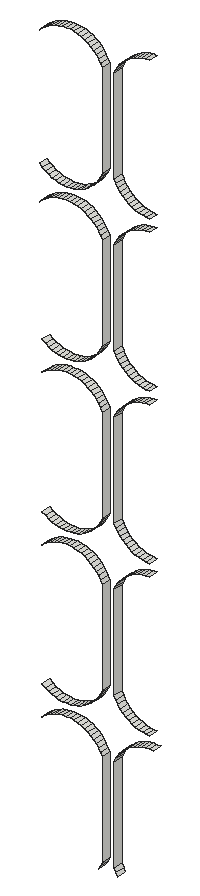
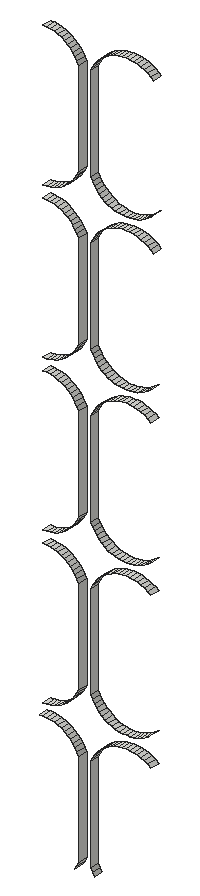
# SketchUp Ruby script. Lengths in inches.
U = 1.inch
M = Sketchup.active_model
def pt(a) = Geom::Point3d.new(a.map { |v| v * U })
def face(e, loops, mat)
  f = e.add_face(loops[0].map { |a| pt(a) })
  loops[1..].each { |l| e.add_face(l.map { |a| pt(a) }).erase! }
  f.material = f.back_material = mat if mat
  f
end
# faces: each face lists its corners as indices into pts; further lists are holes
def faces(e, pts, list, mat = nil) = list.each { |f| face(e, (f[0].is_a?(Array) ? f : [f]).map { |l| l.map { |i| pts[i] } }, mat) }
# xy, xz, yz: faces in a plane at the given z, y or x. An outline is a flat list of corners, or four numbers for a rectangle; further outlines are holes
def ring(l) = l.size == 4 ? [[l[0], l[1]], [l[2], l[1]], [l[2], l[3]], [l[0], l[3]]] : l.each_slice(2).to_a
def flat(e, list, mat, &to3) = list.each { |f| face(e, (f[0].is_a?(Array) ? f : [f]).map { |l| ring(l).map { |u, v| to3.(u, v) } }, mat) }
def xy(e, z, list, mat = nil) = flat(e, list, mat) { |x, y| [x, y, z] }
def xz(e, y, list, mat = nil) = flat(e, list, mat) { |x, z| [x, y, z] }
def yz(e, x, list, mat = nil) = flat(e, list, mat) { |y, z| [x, y, z] }
def lines(e, pts, list) = list.each { |a, b| e.add_line(pt(pts[a]), pt(pts[b])) }
# prism: a flat outline (further loops are holes) pulled along v
def prism(e, loops, v, mat = nil)
  f = face(e, loops, mat); d = Geom::Vector3d.new(v.map { |x| x * U })
  f.pushpull(f.normal.samedirection?(d) ? d.length : -d.length)
end
def box(e, o, s, mat = nil) = prism(e, [[o, [o[0] + s[0], o[1], o[2]], [o[0] + s[0], o[1] + s[1], o[2]], [o[0], o[1] + s[1], o[2]]]], [0, 0, s[2]], mat)
def at(x, y, z, deg = 0) = Geom::Transformation.translation(pt([x, y, z])) * Geom::Transformation.rotation(ORIGIN, Z_AXIS, deg.degrees)
def axes(o, x, y, z) = Geom::Transformation.new([*x, 0, *y, 0, *z, 0, *pt(o).to_a, 1])
def part(name) = M.definitions.add(name)
# library, detail: a bought-in or finely detailed component or shape, given as its bounding box
def library(name, o, s) = part(name).tap { |d| box(d.entities, o, s) }
def detail(e, o, s) = box(e.add_group.entities, o, s)
def put(e, d, t, mat = nil) = e.add_instance(d, t).tap { |i| i.material = mat if mat }
def group(e, t, mat = nil) = e.add_group.tap { |g| g.transformation = t; g.material = mat if mat }.entities
root = M.entities
yz(root,71.5,[[138,52,138.79,60],[138,65,138.79,73],[138,78,138.79,86],[138,91,138.79,99],[138,104,138.79,112]])
yz(root,72.5,[[138,52,138.79,60],[138,65,138.79,73],[138,78,138.79,86],[138,91,138.79,99],[138,104,138.79,112]])
p = [[71.36,138.79,51.71],[71.2,138.79,51.44],[71.2,138,51.44],[71.36,138,51.71],[72.8,138.79,51.44],[72.64,138.79,51.71],
  [72.64,138,51.71],[72.8,138,51.44],[71.5,138.79,52],[71.5,138,52],[72.5,138.79,52],[72.5,138,52],
  [71.36,138.79,60.29],[71.5,138.79,60],[71.5,138,60],[71.36,138,60.29],[72.5,138.79,60],[72.64,138.79,60.29],
  [72.64,138,60.29],[72.5,138,60],[71.2,138.79,60.56],[71.2,138,60.56],[72.8,138.79,60.56],[72.8,138,60.56],
  [71.01,138.79,60.82],[71.01,138,60.82],[72.99,138.79,60.82],[72.99,138,60.82],[70.79,138.79,61.05],[70.79,138,61.05],
  [73.21,138.79,61.05],[73.21,138,61.05],[70.56,138.79,61.26],[70.56,138,61.26],[73.44,138.79,61.26],[73.44,138,61.26],
  [66.44,138.79,61.26],[66.7,138.79,61.45],[66.7,138,61.45],[66.44,138,61.26],[70.3,138.79,61.45],[70.3,138,61.45],
  [73.7,138.79,61.45],[73.7,138,61.45],[66.97,138.79,61.62],[66.97,138,61.62],[70.03,138.79,61.62],[70.03,138,61.62],
  [73.97,138.79,61.62],[73.97,138,61.62],[67.26,138.79,61.75],[67.26,138,61.75],[69.74,138.79,61.75],[69.74,138,61.75],
  [74.26,138.79,61.75],[74.26,138,61.75],[67.56,138.79,61.86],[67.56,138,61.86],[69.44,138.79,61.86],[69.44,138,61.86],
  [74.56,138.79,61.86],[74.56,138,61.86],[67.87,138.79,61.9375],[67.87,138,61.9375],[68.18,138.79,61.98],[68.18,138,61.98],
  [68.82,138.79,61.98],[69.13,138.79,61.9375],[69.13,138,61.9375],[68.82,138,61.98],[74.87,138.79,61.9375],[74.87,138,61.9375],
  [75.18,138.79,61.98],[75.18,138,61.98],[68.5,138.79,62],[68.5,138,62],[75.5,138.79,62],[75.5,138,62],
  [75.82,138.79,61.98],[75.82,138,61.98],[68.18,138.79,63.02],[67.87,138.79,63.0625],[67.87,138,63.0625],[68.18,138,63.02],
  [68.5,138.79,63],[68.5,138,63],[68.82,138.79,63.02],[68.82,138,63.02],[69.13,138.79,63.0625],[69.13,138,63.0625],
  [75.18,138.79,63.02],[74.87,138.79,63.0625],[74.87,138,63.0625],[75.18,138,63.02],[75.5,138.79,63],[75.5,138,63],
  [67.56,138.79,63.14],[67.26,138.79,63.25],[67.26,138,63.25],[67.56,138,63.14],[69.44,138.79,63.14],[69.44,138,63.14],
  [69.74,138.79,63.25],[69.74,138,63.25],[74.56,138.79,63.14],[74.26,138.79,63.25],[74.26,138,63.25],[74.56,138,63.14],
  [66.97,138.79,63.38],[66.97,138,63.38],[70.03,138.79,63.38],[70.03,138,63.38],[73.97,138.79,63.38],[73.97,138,63.38],
  [66.7,138.79,63.55],[66.7,138,63.55],[70.3,138.79,63.55],[70.3,138,63.55],[73.7,138.79,63.55],[73.7,138,63.55],
  [66.44,138.79,63.74],[66.44,138,63.74],[70.56,138.79,63.74],[70.56,138,63.74],[73.44,138.79,63.74],[73.44,138,63.74],
  [70.79,138.79,63.95],[70.79,138,63.95],[73.21,138.79,63.95],[73.21,138,63.95],[71.01,138.79,64.18],[71.01,138,64.18],
  [72.99,138.79,64.18],[72.99,138,64.18],[71.2,138.79,64.44],[71.2,138,64.44],[72.8,138.79,64.44],[72.8,138,64.44],
  [71.36,138.79,64.71],[71.36,138,64.71],[72.64,138.79,64.71],[72.64,138,64.71],[71.5,138.79,65],[71.5,138,65],
  [72.5,138.79,65],[72.5,138,65],[71.36,138.79,73.29],[71.5,138.79,73],[71.5,138,73],[71.36,138,73.29],
  [72.5,138.79,73],[72.64,138.79,73.29],[72.64,138,73.29],[72.5,138,73],[71.2,138.79,73.56],[71.2,138,73.56],
  [72.8,138.79,73.56],[72.8,138,73.56],[71.01,138.79,73.82],[71.01,138,73.82],[72.99,138.79,73.82],[72.99,138,73.82],
  [70.79,138.79,74.05],[70.79,138,74.05],[73.21,138.79,74.05],[73.21,138,74.05],[70.56,138.79,74.26],[70.56,138,74.26],
  [73.44,138.79,74.26],[73.44,138,74.26],[66.44,138.79,74.26],[66.7,138.79,74.45],[66.7,138,74.45],[66.44,138,74.26],
  [70.3,138.79,74.45],[70.3,138,74.45],[73.7,138.79,74.45],[73.7,138,74.45],[66.97,138.79,74.62],[66.97,138,74.62],
  [70.03,138.79,74.62],[70.03,138,74.62],[73.97,138.79,74.62],[73.97,138,74.62],[67.26,138.79,74.75],[67.26,138,74.75],
  [69.74,138.79,74.75],[69.74,138,74.75],[74.26,138.79,74.75],[74.26,138,74.75],[67.56,138.79,74.86],[67.56,138,74.86],
  [69.44,138.79,74.86],[69.44,138,74.86],[74.56,138.79,74.86],[74.56,138,74.86],[67.87,138.79,74.9375],[67.87,138,74.9375],
  [68.18,138.79,74.98],[68.18,138,74.98],[68.82,138.79,74.98],[69.13,138.79,74.9375],[69.13,138,74.9375],[68.82,138,74.98],
  [74.87,138.79,74.9375],[74.87,138,74.9375],[75.18,138.79,74.98],[75.18,138,74.98],[68.5,138.79,75],[68.5,138,75],
  [75.5,138.79,75],[75.5,138,75],[68.18,138.79,76.02],[67.87,138.79,76.0625],[67.87,138,76.0625],[68.18,138,76.02],
  [68.5,138.79,76],[68.5,138,76],[68.82,138.79,76.02],[68.82,138,76.02],[69.13,138.79,76.0625],[69.13,138,76.0625],
  [75.18,138.79,76.02],[74.87,138.79,76.0625],[74.87,138,76.0625],[75.18,138,76.02],[75.5,138.79,76],[75.5,138,76],
  [67.56,138.79,76.14],[67.26,138.79,76.25],[67.26,138,76.25],[67.56,138,76.14],[69.44,138.79,76.14],[69.44,138,76.14],
  [69.74,138.79,76.25],[69.74,138,76.25],[74.56,138.79,76.14],[74.26,138.79,76.25],[74.26,138,76.25],[74.56,138,76.14],
  [66.97,138.79,76.38],[66.97,138,76.38],[70.03,138.79,76.38],[70.03,138,76.38],[73.97,138.79,76.38],[73.97,138,76.38],
  [66.7,138.79,76.55],[66.7,138,76.55],[70.3,138.79,76.55],[70.3,138,76.55],[73.7,138.79,76.55],[73.7,138,76.55],
  [66.44,138.79,76.74],[66.44,138,76.74],[70.56,138.79,76.74],[70.56,138,76.74],[73.44,138.79,76.74],[73.44,138,76.74],
  [70.79,138.79,76.95],[70.79,138,76.95],[73.21,138.79,76.95],[73.21,138,76.95],[71.01,138.79,77.18],[71.01,138,77.18],
  [72.99,138.79,77.18],[72.99,138,77.18],[71.2,138.79,77.44],[71.2,138,77.44],[72.8,138.79,77.44],[72.8,138,77.44],
  [71.36,138.79,77.71],[71.36,138,77.71],[72.64,138.79,77.71],[72.64,138,77.71],[71.5,138.79,78],[71.5,138,78],
  [72.5,138.79,78],[72.5,138,78],[71.36,138.79,86.29],[71.5,138.79,86],[71.5,138,86],[71.36,138,86.29],
  [72.5,138.79,86],[72.64,138.79,86.29],[72.64,138,86.29],[72.5,138,86],[71.2,138.79,86.56],[71.2,138,86.56],
  [72.8,138.79,86.56],[72.8,138,86.56],[71.01,138.79,86.82],[71.01,138,86.82],[72.99,138.79,86.82],[72.99,138,86.82],
  [70.79,138.79,87.05],[70.79,138,87.05],[73.21,138.79,87.05],[73.21,138,87.05],[70.56,138.79,87.26],[70.56,138,87.26],
  [73.44,138.79,87.26],[73.44,138,87.26],[66.44,138.79,87.26],[66.7,138.79,87.45],[66.7,138,87.45],[66.44,138,87.26],
  [70.3,138.79,87.45],[70.3,138,87.45],[73.7,138.79,87.45],[73.7,138,87.45],[66.97,138.79,87.62],[66.97,138,87.62],
  [70.03,138.79,87.62],[70.03,138,87.62],[73.97,138.79,87.62],[73.97,138,87.62],[67.26,138.79,87.75],[67.26,138,87.75],
  [69.74,138.79,87.75],[69.74,138,87.75],[74.26,138.79,87.75],[74.26,138,87.75],[67.56,138.79,87.86],[67.56,138,87.86],
  [69.44,138.79,87.86],[69.44,138,87.86],[74.56,138.79,87.86],[74.56,138,87.86],[67.87,138.79,87.9375],[67.87,138,87.9375],
  [68.18,138.79,87.98],[68.18,138,87.98],[68.82,138.79,87.98],[69.13,138.79,87.9375],[69.13,138,87.9375],[68.82,138,87.98],
  [74.87,138.79,87.9375],[74.87,138,87.9375],[75.18,138.79,87.98],[75.18,138,87.98],[68.5,138.79,88],[68.5,138,88],
  [75.5,138.79,88],[75.5,138,88],[68.18,138.79,89.02],[67.87,138.79,89.0625],[67.87,138,89.0625],[68.18,138,89.02],
  [68.5,138.79,89],[68.5,138,89],[68.82,138.79,89.02],[68.82,138,89.02],[69.13,138.79,89.0625],[69.13,138,89.0625],
  [75.18,138.79,89.02],[74.87,138.79,89.0625],[74.87,138,89.0625],[75.18,138,89.02],[75.5,138.79,89],[75.5,138,89],
  [67.56,138.79,89.14],[67.26,138.79,89.25],[67.26,138,89.25],[67.56,138,89.14],[69.44,138.79,89.14],[69.44,138,89.14],
  [69.74,138.79,89.25],[69.74,138,89.25],[74.56,138.79,89.14],[74.26,138.79,89.25],[74.26,138,89.25],[74.56,138,89.14],
  [66.97,138.79,89.38],[66.97,138,89.38],[70.03,138.79,89.38],[70.03,138,89.38],[73.97,138.79,89.38],[73.97,138,89.38],
  [66.7,138.79,89.55],[66.7,138,89.55],[70.3,138.79,89.55],[70.3,138,89.55],[73.7,138.79,89.55],[73.7,138,89.55],
  [66.44,138.79,89.74],[66.44,138,89.74],[70.56,138.79,89.74],[70.56,138,89.74],[73.44,138.79,89.74],[73.44,138,89.74],
  [70.79,138.79,89.95],[70.79,138,89.95],[73.21,138.79,89.95],[73.21,138,89.95],[71.01,138.79,90.18],[71.01,138,90.18],
  [72.99,138.79,90.18],[72.99,138,90.18],[71.2,138.79,90.44],[71.2,138,90.44],[72.8,138.79,90.44],[72.8,138,90.44],
  [71.36,138.79,90.71],[71.36,138,90.71],[72.64,138.79,90.71],[72.64,138,90.71],[71.5,138.79,91],[71.5,138,91],
  [72.5,138.79,91],[72.5,138,91],[71.36,138.79,99.29],[71.5,138.79,99],[71.5,138,99],[71.36,138,99.29],
  [72.5,138.79,99],[72.64,138.79,99.29],[72.64,138,99.29],[72.5,138,99],[71.2,138.79,99.56],[71.2,138,99.56],
  [72.8,138.79,99.56],[72.8,138,99.56],[71.01,138.79,99.82],[71.01,138,99.82],[72.99,138.79,99.82],[72.99,138,99.82],
  [70.79,138.79,100.05],[70.79,138,100.05],[73.21,138.79,100.05],[73.21,138,100.05],[66.21,138.79,100.05],[66.44,138.79,100.26],
  [66.44,138,100.26],[66.21,138,100.05],[70.56,138.79,100.26],[70.56,138,100.26],[73.44,138.79,100.26],[73.44,138,100.26],
  [66.7,138.79,100.45],[66.7,138,100.45],[70.3,138.79,100.45],[70.3,138,100.45],[73.7,138.79,100.45],[73.7,138,100.45],
  [66.97,138.79,100.62],[66.97,138,100.62],[70.03,138.79,100.62],[70.03,138,100.62],[73.97,138.79,100.62],[73.97,138,100.62],
  [67.26,138.79,100.75],[67.26,138,100.75],[69.74,138.79,100.75],[69.74,138,100.75],[74.26,138.79,100.75],[74.26,138,100.75],
  [67.56,138.79,100.86],[67.56,138,100.86],[69.44,138.79,100.86],[69.44,138,100.86],[74.56,138.79,100.86],[74.56,138,100.86],
  [67.87,138.79,100.9375],[67.87,138,100.9375],[68.18,138.79,100.98],[68.18,138,100.98],[68.82,138.79,100.98],[69.13,138.79,100.9375],
  [69.13,138,100.9375],[68.82,138,100.98],[74.87,138.79,100.9375],[74.87,138,100.9375],[75.18,138.79,100.98],[75.18,138,100.98],
  [68.5,138.79,101],[68.5,138,101],[75.5,138.79,101],[75.5,138,101],[68.18,138.79,102.02],[67.87,138.79,102.0625],
  [67.87,138,102.0625],[68.18,138,102.02],[68.5,138.79,102],[68.5,138,102],[68.82,138.79,102.02],[68.82,138,102.02],
  [69.13,138.79,102.0625],[69.13,138,102.0625],[75.18,138.79,102.02],[74.87,138.79,102.0625],[74.87,138,102.0625],[75.18,138,102.02],
  [75.5,138.79,102],[75.5,138,102],[67.56,138.79,102.14],[67.26,138.79,102.25],[67.26,138,102.25],[67.56,138,102.14],
  [69.44,138.79,102.14],[69.44,138,102.14],[69.74,138.79,102.25],[69.74,138,102.25],[74.56,138.79,102.14],[74.26,138.79,102.25],
  [74.26,138,102.25],[74.56,138,102.14],[66.97,138.79,102.38],[66.97,138,102.38],[70.03,138.79,102.38],[70.03,138,102.38],
  [73.97,138.79,102.38],[73.97,138,102.38],[66.7,138.79,102.55],[66.7,138,102.55],[70.3,138.79,102.55],[70.3,138,102.55],
  [73.7,138.79,102.55],[73.7,138,102.55],[66.44,138.79,102.74],[66.44,138,102.74],[70.56,138.79,102.74],[70.56,138,102.74],
  [73.44,138.79,102.74],[73.44,138,102.74],[66.21,138.79,102.95],[66.21,138,102.95],[70.79,138.79,102.95],[70.79,138,102.95],
  [73.21,138.79,102.95],[73.21,138,102.95],[71.01,138.79,103.18],[71.01,138,103.18],[72.99,138.79,103.18],[72.99,138,103.18],
  [71.2,138.79,103.44],[71.2,138,103.44],[72.8,138.79,103.44],[72.8,138,103.44],[71.36,138.79,103.71],[71.36,138,103.71],
  [72.64,138.79,103.71],[72.64,138,103.71],[71.5,138.79,104],[71.5,138,104],[72.5,138.79,104],[72.5,138,104],
  [71.36,138.79,112.29],[71.5,138.79,112],[71.5,138,112],[71.36,138,112.29],[72.5,138.79,112],[72.64,138.79,112.29],
  [72.64,138,112.29],[72.5,138,112],[71.2,138.79,112.56],[71.2,138,112.56],[72.8,138.79,112.56],[72.8,138,112.56],
  [71.01,138.79,112.82],[71.01,138,112.82],[72.99,138.79,112.82],[72.99,138,112.82],[70.79,138.79,113.05],[70.79,138,113.05],
  [73.21,138.79,113.05],[73.21,138,113.05],[66.21,138.79,113.05],[66.44,138.79,113.26],[66.44,138,113.26],[66.21,138,113.05],
  [70.56,138.79,113.26],[70.56,138,113.26],[73.44,138.79,113.26],[73.44,138,113.26],[66.7,138.79,113.45],[66.7,138,113.45],
  [70.3,138.79,113.45],[70.3,138,113.45],[73.7,138.79,113.45],[73.7,138,113.45],[66.97,138.79,113.62],[66.97,138,113.62],
  [70.03,138.79,113.62],[70.03,138,113.62],[73.97,138.79,113.62],[73.97,138,113.62],[67.26,138.79,113.75],[67.26,138,113.75],
  [69.74,138.79,113.75],[69.74,138,113.75],[74.26,138.79,113.75],[74.26,138,113.75],[67.56,138.79,113.86],[67.56,138,113.86],
  [69.44,138.79,113.86],[69.44,138,113.86],[74.56,138.79,113.86],[74.56,138,113.86],[67.87,138.79,113.9375],[67.87,138,113.9375],
  [68.18,138.79,113.98],[68.18,138,113.98],[68.82,138.79,113.98],[69.13,138.79,113.9375],[69.13,138,113.9375],[68.82,138,113.98],
  [74.87,138.79,113.9375],[74.87,138,113.9375],[75.18,138.79,113.98],[75.18,138,113.98],[68.5,138.79,114],[68.5,138,114],
  [75.5,138.79,114],[75.5,138,114]]
faces(root,p,[[0,1,2,3],[4,5,6,7],[8,0,3,9],[5,10,11,6],[12,13,14,15],[16,17,18,19],[20,12,15,21],[17,22,23,18],
  [24,20,21,25],[22,26,27,23],[28,24,25,29],[26,30,31,27],[32,28,29,33],[30,34,35,31],[36,37,38,39],[40,32,33,41],
  [34,42,43,35],[37,44,45,38],[46,40,41,47],[42,48,49,43],[44,50,51,45],[52,46,47,53],[48,54,55,49],[50,56,57,51],
  [58,52,53,59],[54,60,61,55],[56,62,63,57],[62,64,65,63],[66,67,68,69],[67,58,59,68],[60,70,71,61],[70,72,73,71],
  [64,74,75,65],[74,66,69,75],[72,76,77,73],[76,78,79,77],[80,81,82,83],[84,80,83,85],[86,84,85,87],[88,86,87,89],
  [90,91,92,93],[94,90,93,95],[96,97,98,99],[81,96,99,82],[100,88,89,101],[102,100,101,103],[104,105,106,107],[91,104,107,92],
  [97,108,109,98],[110,102,103,111],[105,112,113,106],[108,114,115,109],[116,110,111,117],[112,118,119,113],[114,120,121,115],[122,116,117,123],
  [118,124,125,119],[126,122,123,127],[124,128,129,125],[130,126,127,131],[128,132,133,129],[134,130,131,135],[132,136,137,133],[138,134,135,139],
  [136,140,141,137],[142,138,139,143],[140,144,145,141],[146,147,148,149],[150,151,152,153],[154,146,149,155],[151,156,157,152],[158,154,155,159],
  [156,160,161,157],[162,158,159,163],[160,164,165,161],[166,162,163,167],[164,168,169,165],[170,171,172,173],[174,166,167,175],[168,176,177,169],
  [171,178,179,172],[180,174,175,181],[176,182,183,177],[178,184,185,179],[186,180,181,187],[182,188,189,183],[184,190,191,185],[192,186,187,193],
  [188,194,195,189],[190,196,197,191],[196,198,199,197],[200,201,202,203],[201,192,193,202],[194,204,205,195],[204,206,207,205],[198,208,209,199],
  [208,200,203,209],[206,210,211,207],[212,213,214,215],[216,212,215,217],[218,216,217,219],[220,218,219,221],[222,223,224,225],[226,222,225,227],
  [228,229,230,231],[213,228,231,214],[232,220,221,233],[234,232,233,235],[236,237,238,239],[223,236,239,224],[229,240,241,230],[242,234,235,243],
  [237,244,245,238],[240,246,247,241],[248,242,243,249],[244,250,251,245],[246,252,253,247],[254,248,249,255],[250,256,257,251],[258,254,255,259],
  [256,260,261,257],[262,258,259,263],[260,264,265,261],[266,262,263,267],[264,268,269,265],[270,266,267,271],[268,272,273,269],[274,270,271,275],
  [272,276,277,273],[278,279,280,281],[282,283,284,285],[286,278,281,287],[283,288,289,284],[290,286,287,291],[288,292,293,289],[294,290,291,295],
  [292,296,297,293],[298,294,295,299],[296,300,301,297],[302,303,304,305],[306,298,299,307],[300,308,309,301],[303,310,311,304],[312,306,307,313],
  [308,314,315,309],[310,316,317,311],[318,312,313,319],[314,320,321,315],[316,322,323,317],[324,318,319,325],[320,326,327,321],[322,328,329,323],
  [328,330,331,329],[332,333,334,335],[333,324,325,334],[326,336,337,327],[336,338,339,337],[330,340,341,331],[340,332,335,341],[338,342,343,339],
  [344,345,346,347],[348,344,347,349],[350,348,349,351],[352,350,351,353],[354,355,356,357],[358,354,357,359],[360,361,362,363],[345,360,363,346],
  [364,352,353,365],[366,364,365,367],[368,369,370,371],[355,368,371,356],[361,372,373,362],[374,366,367,375],[369,376,377,370],[372,378,379,373],
  [380,374,375,381],[376,382,383,377],[378,384,385,379],[386,380,381,387],[382,388,389,383],[390,386,387,391],[388,392,393,389],[394,390,391,395],
  [392,396,397,393],[398,394,395,399],[396,400,401,397],[402,398,399,403],[400,404,405,401],[406,402,403,407],[404,408,409,405],[410,411,412,413],
  [414,415,416,417],[418,410,413,419],[415,420,421,416],[422,418,419,423],[420,424,425,421],[426,422,423,427],[424,428,429,425],[430,431,432,433],
  [434,426,427,435],[428,436,437,429],[431,438,439,432],[440,434,435,441],[436,442,443,437],[438,444,445,439],[446,440,441,447],[442,448,449,443],
  [444,450,451,445],[452,446,447,453],[448,454,455,449],[450,456,457,451],[458,452,453,459],[454,460,461,455],[456,462,463,457],[462,464,465,463],
  [466,467,468,469],[467,458,459,468],[460,470,471,461],[470,472,473,471],[464,474,475,465],[474,466,469,475],[472,476,477,473],[478,479,480,481],
  [482,478,481,483],[484,482,483,485],[486,484,485,487],[488,489,490,491],[492,488,491,493],[494,495,496,497],[479,494,497,480],[498,486,487,499],
  [500,498,499,501],[502,503,504,505],[489,502,505,490],[495,506,507,496],[508,500,501,509],[503,510,511,504],[506,512,513,507],[514,508,509,515],
  [510,516,517,511],[512,518,519,513],[520,514,515,521],[516,522,523,517],[518,524,525,519],[526,520,521,527],[522,528,529,523],[530,526,527,531],
  [528,532,533,529],[534,530,531,535],[532,536,537,533],[538,534,535,539],[536,540,541,537],[542,538,539,543],[540,544,545,541],[546,547,548,549],
  [550,551,552,553],[554,546,549,555],[551,556,557,552],[558,554,555,559],[556,560,561,557],[562,558,559,563],[560,564,565,561],[566,567,568,569],
  [570,562,563,571],[564,572,573,565],[567,574,575,568],[576,570,571,577],[572,578,579,573],[574,580,581,575],[582,576,577,583],[578,584,585,579],
  [580,586,587,581],[588,582,583,589],[584,590,591,585],[586,592,593,587],[594,588,589,595],[590,596,597,591],[592,598,599,593],[598,600,601,599],
  [602,603,604,605],[603,594,595,604],[596,606,607,597],[606,608,609,607],[600,610,611,601],[610,602,605,611],[608,612,613,609]])
